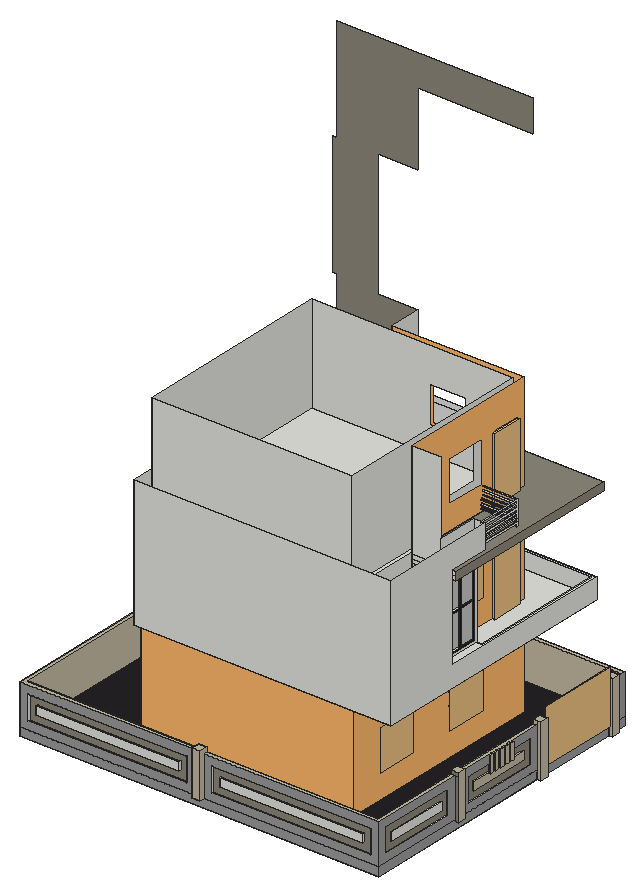
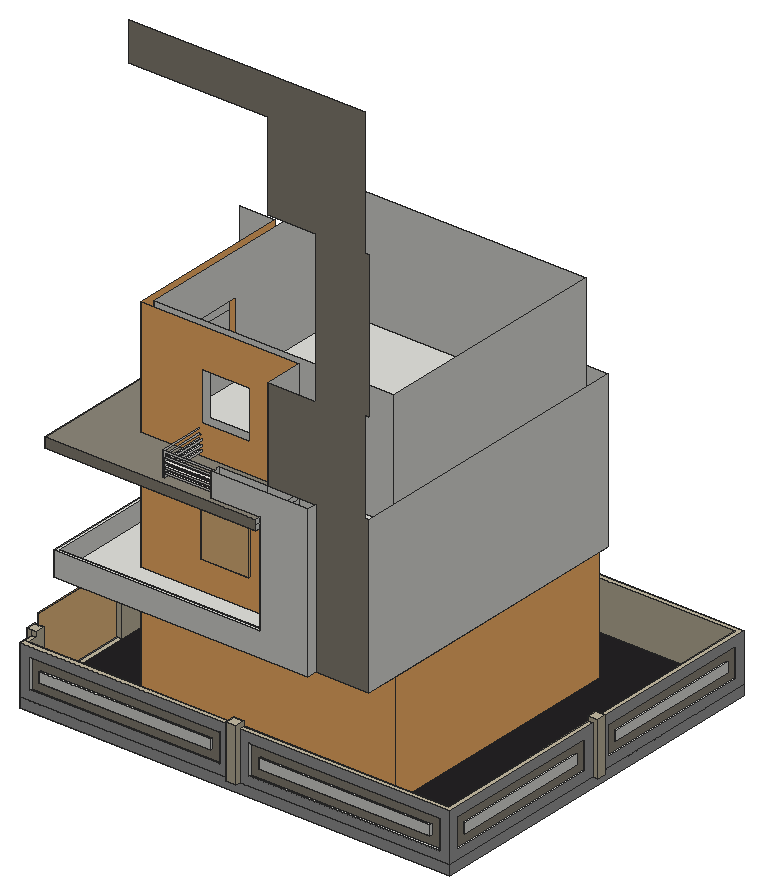
# SketchUp Ruby script. Lengths in inches.
U = 1.inch
M = Sketchup.active_model
def pt(a) = Geom::Point3d.new(a.map { |v| v * U })
def face(e, loops, mat)
  f = e.add_face(loops[0].map { |a| pt(a) })
  loops[1..].each { |l| e.add_face(l.map { |a| pt(a) }).erase! }
  f.material = f.back_material = mat if mat
  f
end
# faces: each face lists its corners as indices into pts; further lists are holes
def faces(e, pts, list, mat = nil) = list.each { |f| face(e, (f[0].is_a?(Array) ? f : [f]).map { |l| l.map { |i| pts[i] } }, mat) }
# xy, xz, yz: faces in a plane at the given z, y or x. An outline is a flat list of corners, or four numbers for a rectangle; further outlines are holes
def ring(l) = l.size == 4 ? [[l[0], l[1]], [l[2], l[1]], [l[2], l[3]], [l[0], l[3]]] : l.each_slice(2).to_a
def flat(e, list, mat, &to3) = list.each { |f| face(e, (f[0].is_a?(Array) ? f : [f]).map { |l| ring(l).map { |u, v| to3.(u, v) } }, mat) }
def xy(e, z, list, mat = nil) = flat(e, list, mat) { |x, y| [x, y, z] }
def xz(e, y, list, mat = nil) = flat(e, list, mat) { |x, z| [x, y, z] }
def yz(e, x, list, mat = nil) = flat(e, list, mat) { |y, z| [x, y, z] }
def lines(e, pts, list) = list.each { |a, b| e.add_line(pt(pts[a]), pt(pts[b])) }
# prism: a flat outline (further loops are holes) pulled along v
def prism(e, loops, v, mat = nil)
  f = face(e, loops, mat); d = Geom::Vector3d.new(v.map { |x| x * U })
  f.pushpull(f.normal.samedirection?(d) ? d.length : -d.length)
end
def box(e, o, s, mat = nil) = prism(e, [[o, [o[0] + s[0], o[1], o[2]], [o[0] + s[0], o[1] + s[1], o[2]], [o[0], o[1] + s[1], o[2]]]], [0, 0, s[2]], mat)
def at(x, y, z, deg = 0) = Geom::Transformation.translation(pt([x, y, z])) * Geom::Transformation.rotation(ORIGIN, Z_AXIS, deg.degrees)
def axes(o, x, y, z) = Geom::Transformation.new([*x, 0, *y, 0, *z, 0, *pt(o).to_a, 1])
def part(name) = M.definitions.add(name)
# library, detail: a bought-in or finely detailed component or shape, given as its bounding box
def library(name, o, s) = part(name).tap { |d| box(d.entities, o, s) }
def detail(e, o, s) = box(e.add_group.entities, o, s)
def put(e, d, t, mat = nil) = e.add_instance(d, t).tap { |i| i.material = mat if mat }
def group(e, t, mat = nil) = e.add_group.tap { |g| g.transformation = t; g.material = mat if mat }.entities
root = M.entities
M.materials.add("Brick_05_1K").color = [255, 185, 107]
M.materials.add("Brick_05_1K1").color = [195, 185, 161]
M.materials.add("Brick_09_1K").color = [135, 129, 110]
M.materials.add("M02_Ash_Whisper").color = [196, 196, 196]
M.materials.add("M08_Obsidian_Black").color = [30, 30, 30]
M.materials.add("Marble_07_1K").color = [36, 34, 36]
M.materials.add("Metal_06_1K").color = [238, 236, 231]
M.materials.add("Plaster_06_1K").color = [141, 135, 122]
M.materials.add("ThomThom - Waistcoat1").color = [155, 155, 155]
c1 = library("Modern+Gate+1",[0,0,0],[118.11,1.97,78.74])
c2 = library("mesh-164",[-1582.71,-3144.16,-23.22],[2366.42,2227.34,65.81])
c3 = part("Group13")
put(c3.entities,c2,at(294.66,859.51,3.5))
c4 = library("porta+4",[0.2,-5.42,1.33],[46.55,4.72,83.21])
xy(root,0,[[6,6,537.31,461.27]])
xy(root,0,[[537.31,299.27,543.31,311.27],[537.31,431.27,543.31,443.27]],"Brick_05_1K1")
xy(root,12,[[129.93,88.15,429.93,388.15]])
xy(root,12,[[265.65,0,277.65,6],[6,6,6,461.27,537.31,461.27,537.31,431.27,531.31,431.27,531.31,455.27,12,455.27,12,12,531.31,12,531.31,311.27,537.31,311.27,537.31,6],[537.31,146.64,543.31,158.64],[0,227.64,6,239.64],[531.31,311.27,537.31,431.27],
  [265.65,461.27,277.65,467.27]],"Brick_05_1K1")
xy(root,12,[[[12,12,531.31,455.27],[123.93,82.15,438.93,397.15]]],"Marble_07_1K")
xy(root,24,[[18,6,253.65,9],[289.65,6,525.31,9],[6,18,9,215.64],[534.31,18,537.31,134.64],[6,251.64,9,449.27],
  [18,458.27,253.65,461.27],[289.65,458.27,525.31,461.27]])
xy(root,24,[[534.31,170.64,537.31,287.27]],"Brick_05_1K1")
xy(root,36,[[30,6,241.65,9],[301.65,6,513.31,9],[6,30,9,203.64],[534.31,30,537.31,122.64],[6,263.64,9,437.27],
  [30,458.27,241.65,461.27],[301.65,458.27,513.31,461.27]])
xy(root,36,[[534.31,182.64,537.31,275.27]],"Brick_05_1K1")
xy(root,47.87,[[537.31,237.93,540.31,242.66],[537.31,247.4,540.31,252.14]],"Brick_05_1K1")
xy(root,48,[[30,6,241.65,9],[301.65,6,513.31,9],[6,30,9,203.64],[534.31,30,537.31,122.64],[6,263.64,9,437.27],
  [30,458.27,241.65,461.27],[301.65,458.27,513.31,461.27]])
xy(root,48,[[534.31,182.64,537.31,275.27],[537.31,209.5,540.31,214.24],[537.31,218.98,540.31,223.71],[537.31,228.45,540.31,233.1875]],"Brick_05_1K1")
xy(root,51,[[429.93,133.15,438.93,187.15],[429.93,262.15,438.93,316.15]])
xy(root,60,[[18,6,253.65,9],[289.65,6,525.31,9],[6,18,9,215.64],[534.31,18,537.31,134.64],[6,251.64,9,449.27],
  [18,458.27,253.65,461.27],[289.65,458.27,525.31,461.27]])
xy(root,60,[[534.31,170.64,537.31,287.27]],"Brick_05_1K1")
xy(root,72,[[6,6,265.65,6,265.65,12,12,12,12,227.64,6,227.64],[277.65,6,537.31,6,537.31,146.64,531.31,146.64,531.31,12,277.65,12],[531.31,158.64,537.31,158.64,537.31,209.5,540.31,209.5,540.31,214.24,537.31,214.24,537.31,218.98,540.31,218.98,540.31,223.71,537.31,223.71,537.31,228.45,540.31,228.45,540.31,233.1875,537.31,233.1875,537.31,237.93,540.31,237.93,540.31,242.66,537.31,242.66,537.31,247.4,540.31,247.4,540.31,252.14,537.31,252.14,537.31,299.27,531.31,299.27],[6,239.64,12,239.64,12,455.27,265.65,455.27,265.65,461.27,6,461.27],[531.31,443.27,537.31,455.27],
  [277.65,455.27,537.31,461.27]],"Brick_05_1K1")
xy(root,78,[[265.65,0,277.65,12],[531.31,146.64,543.31,158.64],[0,227.64,12,239.64],[531.31,299.27,543.31,311.27],[531.31,431.27,543.31,443.27],
  [265.65,455.27,277.65,467.27]],"Brick_05_1K1")
xy(root,105,[[429.93,133.15,438.93,187.15],[429.93,262.15,438.93,316.15]])
xy(root,156,[[117.93,76.15,117.93,82.15,438.93,82.15,438.93,397.15,117.93,397.15,117.93,445.15,183.93,445.15,183.93,457.15,498.93,457.15,498.93,76.15],[117.93,82.15,123.93,88.15],[123.93,82.15,438.93,88.15],[117.93,88.15,123.93,397.15],[123.93,88.15,129.93,397.15],
  [129.93,88.15,429.93,388.15],[429.93,88.15,438.93,397.15],[129.93,388.15,429.93,397.15]])
xy(root,162,[[132.93,91.15,429.93,388.15],[438.93,190.15,482.43,190.15,482.43,250.15,494.43,250.15,494.43,452.65,243.93,452.65,243.93,397.15,438.93,397.15]])
xy(root,165,[[429.93,346.15,438.93,382.15]])
xy(root,186,[[486.93,190.15,498.93,190.15,498.93,457.15,243.93,457.15,243.93,452.65,494.43,452.65,494.43,250.15,486.93,250.15]])
xy(root,192,[[484.46,196.15,486.93,219.15],[484.46,221.15,486.93,244.15]])
xy(root,201,[[429.93,262.15,438.93,316.15],[306.93,388.15,360.93,397.15]])
xy(root,243,[[484.46,196.15,486.93,219.15],[484.46,221.15,486.93,244.15]])
xy(root,245,[[484.46,196.15,486.93,219.15],[484.46,221.15,486.93,244.15]])
xy(root,255,[[429.93,262.15,438.93,316.15],[429.93,346.15,438.93,382.15],[306.93,388.15,360.93,397.15]])
xy(root,294,[[484.46,196.15,486.93,219.15],[484.46,221.15,486.93,244.15]])
xy(root,300,[[438.93,190.15,438.93,397.15,243.93,397.15,243.93,463.15,504.93,463.15,504.93,190.15,486.93,190.15,486.93,250.15,482.43,250.15,482.43,190.15]],"Plaster_06_1K")
xy(root,306,[[132.93,91.15,429.93,388.15]])
xy(root,312,[[132.93,91.15,429.93,388.15],[482.43,190.15,498.93,250.15],[491.43,317.65,492.93,319.15],[243.93,445.15,303.93,457.15],[363.93,449.15,366.93,453.15]])
xy(root,312,[[[438.93,190.15,482.43,190.15,482.43,250.15,498.93,250.15,498.93,190.15,504.93,190.15,504.93,463.15,243.93,463.15,243.93,457.15,303.93,457.15,303.93,445.15,243.93,445.15,243.93,397.15,438.93,397.15],[363.93,449.15,366.93,453.15],[491.43,317.65,492.93,319.15]]],"Plaster_06_1K")
xy(root,315,[[429.93,346.15,438.93,379.15],[429.93,379.15,438.93,382.15]])
xy(root,316,[[363.93,397.1,366.93,449.15],[303.93,449.15,363.93,453.15]])
xy(root,316,[[491.43,250.15,492.93,317.65],[438.93,317.65,491.43,319.15]],"Metal_06_1K")
xy(root,318,[[491.43,250.15,492.93,317.65],[438.93,317.65,491.43,319.15],[363.93,397.1,366.93,449.15],[303.93,449.15,363.93,453.15]],"Metal_06_1K")
xy(root,322,[[491.43,250.15,492.93,317.65],[438.93,317.65,491.43,319.15],[363.93,397.1,366.93,449.15],[303.93,449.15,363.93,453.15]])
xy(root,324,[[491.43,250.15,492.93,317.65],[438.93,317.65,491.43,319.15],[363.93,397.1,366.93,449.15],[303.93,449.15,363.93,453.15]],"Metal_06_1K")
xy(root,328,[[491.43,250.15,492.93,317.65],[438.93,317.65,491.43,319.15],[363.93,397.1,366.93,449.15],[303.93,449.15,363.93,453.15]])
xy(root,330,[[491.43,250.15,492.93,317.65],[438.93,317.65,491.43,319.15],[363.93,397.1,366.93,449.15],[303.93,449.15,363.93,453.15]],"Metal_06_1K")
xz(root,0,[[265.65,12,277.65,78]],"Brick_05_1K1")
xz(root,6,[[30,36,241.65,48],[301.65,36,513.31,48]])
xz(root,6,[[6,0,537.31,12],[[6,12,265.65,72],[18,24,253.65,60]],[[277.65,12,537.31,72],[289.65,24,525.31,60]]],"ThomThom - Waistcoat1")
xz(root,9,[[[18,24,253.65,60],[30,36,241.65,48]],[[289.65,24,525.31,60],[301.65,36,513.31,48]]],"Plaster_06_1K")
xz(root,12,[[12,12,12,72,265.65,72,265.65,78,277.65,78,277.65,72,531.31,72,531.31,12]],"Brick_05_1K1")
xz(root,18,[[6,24,9,60],[534.31,24,537.31,60]])
xz(root,30,[[6,36,9,48],[534.31,36,537.31,48]])
xz(root,76.15,[[117.93,156,498.93,348]])
xz(root,82.15,[[123.93,12,438.93,156]],"Brick_05_1K")
xz(root,88.15,[[129.93,12,429.93,156]])
xz(root,91.15,[[132.93,162,429.93,306],[132.93,312,429.93,456]])
xz(root,122.64,[[534.31,36,537.31,48]])
xz(root,133.15,[[429.93,51,438.93,105]])
xz(root,134.64,[[534.31,24,537.31,60]])
xz(root,146.64,[[537.31,12,543.31,72],[531.31,72,543.31,78]],"Brick_09_1K")
xz(root,158.64,[[537.31,12,543.31,72],[531.31,72,543.31,78]],"Brick_09_1K")
xz(root,170.64,[[534.31,24,537.31,60]],"Brick_05_1K1")
xz(root,182.64,[[534.31,36,537.31,48]],"Brick_05_1K1")
xz(root,187.15,[[429.93,51,438.93,105]])
xz(root,190.15,[[438.93,162,482.43,300],[482.43,186,482.43,300,438.93,300,438.93,306,498.93,306,498.93,300,486.93,300,486.93,186],[486.93,186,498.93,300],[498.93,300,504.93,306],[438.93,306,498.93,312],
  [498.93,306,504.93,312],[438.93,312,482.43,456]])
xz(root,196.15,[[484.46,192,486.93,243],[484.46,245,486.93,294]])
xz(root,203.64,[[6,36,9,48]])
xz(root,209.5,[[537.31,48,540.31,72]],"Brick_05_1K1")
xz(root,214.24,[[537.31,48,540.31,72]],"Brick_05_1K1")
xz(root,215.64,[[6,24,9,60]])
xz(root,218.98,[[537.31,48,540.31,72]],"Brick_05_1K1")
xz(root,219.15,[[484.46,192,486.93,243],[484.46,245,486.93,294]])
xz(root,221.15,[[484.46,192,486.93,243],[484.46,245,486.93,294]])
xz(root,223.71,[[537.31,48,540.31,72]],"Brick_05_1K1")
xz(root,227.64,[[0,12,6,12,6,72,12,72,12,78,0,78]],"Brick_05_1K1")
xz(root,228.45,[[537.31,48,540.31,72]],"Brick_05_1K1")
xz(root,233.1875,[[537.31,48,540.31,72]],"Brick_05_1K1")
xz(root,237.93,[[537.31,47.87,540.31,72]],"Brick_05_1K1")
xz(root,239.64,[[0,12,0,78,12,78,12,72,6,72,6,12]],"Brick_05_1K1")
xz(root,242.66,[[537.31,47.87,540.31,72]],"Brick_05_1K1")
xz(root,244.15,[[484.46,192,486.93,243],[484.46,245,486.93,294]])
xz(root,247.4,[[537.31,47.87,540.31,72]],"Brick_05_1K1")
xz(root,250.15,[[482.43,162,482.43,300,486.93,300,486.93,186,494.43,186,494.43,162],[[482.43,312,482.43,348,491.43,348,491.43,346,492.93,346,492.93,348,498.93,348,498.93,312],[491.43,340,492.93,342],[491.43,334,492.93,336],[491.43,328,492.93,330],[491.43,322,492.93,324]],[491.43,322,492.93,324],[491.43,328,492.93,330]])
xz(root,250.15,[[491.43,316,492.93,318]],"Metal_06_1K")
xz(root,251.64,[[6,24,9,60]])
xz(root,252.14,[[537.31,47.87,540.31,72]],"Brick_05_1K1")
xz(root,262.15,[[429.93,51,438.93,105],[429.93,201,438.93,255]])
xz(root,263.64,[[6,36,9,48]])
xz(root,275.27,[[534.31,36,537.31,48]],"Brick_05_1K1")
xz(root,287.27,[[534.31,24,537.31,60]],"Brick_05_1K1")
xz(root,299.27,[[537.31,0,543.31,78],[531.31,72,537.31,78]],"Brick_05_1K1")
xz(root,311.27,[[537.31,0,537.31,12,531.31,12,531.31,78,543.31,78,543.31,0]],"Brick_05_1K1")
xz(root,316.15,[[429.93,51,438.93,105],[429.93,201,438.93,255]])
xz(root,317.65,[[491.43,312,492.93,316],[491.43,318,492.93,322],[491.43,322,492.93,324],[491.43,324,492.93,328],[491.43,330,492.93,334]])
xz(root,317.65,[[438.93,316,491.43,318],[438.93,322,491.43,324],[438.93,328,491.43,330]],"Metal_06_1K")
xz(root,319.15,[[491.43,312,492.93,318],[438.93,316,491.43,318],[491.43,318,491.43,328,438.93,328,438.93,330,491.43,330,491.43,334,438.93,334,438.93,336,491.43,336,491.43,340,438.93,340,438.93,342,491.43,342,491.43,346,438.93,346,438.93,348,492.93,348,492.93,318],[438.93,322,491.43,324]],"Metal_06_1K")
xz(root,346.15,[[429.93,165,438.93,255],[429.93,315,438.93,405]])
xz(root,382.15,[[429.93,165,438.93,255],[429.93,315,438.93,405]])
xz(root,388.15,[[129.93,12,429.93,156],[[132.93,162,429.93,306],[306.93,201,360.93,255]],[[132.93,312,429.93,456],[306.93,351,360.93,405]]])
xz(root,397.1,[[363.93,316,366.93,318],[363.93,322,366.93,324],[363.93,328,366.93,330]])
xz(root,397.15,[[243.93,300,438.93,306]])
xz(root,397.15,[[123.93,12,438.93,156],[[243.93,162,438.93,300],[303.93,198,363.93,258]],[[303.93,198,363.93,258],[306.93,201,360.93,255]],[[243.93,312,438.93,456],[303.93,348,363.93,408],[363.93,340,366.93,342],[363.93,334,366.93,336]]],"Brick_05_1K")
xz(root,431.27,[[537.31,0,543.31,0,543.31,78,531.31,78,531.31,12,537.31,12]],"Brick_05_1K1")
xz(root,437.27,[[6,36,9,48]])
xz(root,443.27,[[537.31,0,543.31,78],[531.31,72,537.31,78]],"Brick_05_1K1")
xz(root,445.15,[[243.93,312,303.93,342]])
xz(root,445.15,[[117.93,156,117.93,348,123.93,348,123.93,462,117.93,462,117.93,642,123.93,642,123.93,798,414.93,798,414.93,750,243.93,750,243.93,642,183.93,642,183.93,456,243.93,456,243.93,342,183.93,342,183.93,156]],"Plaster_06_1K")
xz(root,449.15,[[363.93,312,366.93,316],[303.93,316,363.93,318],[363.93,318,366.93,322],[303.93,322,363.93,324],[363.93,324,366.93,328],
  [303.93,328,363.93,330],[363.93,330,366.93,334]])
xz(root,449.27,[[6,24,9,60]])
xz(root,452.65,[[243.93,162,494.43,186]])
xz(root,453.15,[[363.93,312,363.93,316,303.93,316,303.93,318,363.93,318,363.93,322,303.93,322,303.93,324,363.93,324,363.93,328,303.93,328,303.93,330,363.93,330,363.93,334,303.93,334,303.93,336,363.93,336,363.93,340,303.93,340,303.93,342,366.93,342,366.93,312]],"Metal_06_1K")
xz(root,455.27,[[12,12,531.31,12,531.31,72,277.65,72,277.65,78,265.65,78,265.65,72,12,72]],"Brick_05_1K1")
xz(root,457.15,[[183.93,156,183.93,342,303.93,342,303.93,312,243.93,312,243.93,186,498.93,186,498.93,156]])
xz(root,458.27,[[[18,24,253.65,60],[30,36,241.65,48]],[[289.65,24,525.31,60],[301.65,36,513.31,48]]],"Plaster_06_1K")
xz(root,461.27,[[30,36,241.65,48],[301.65,36,513.31,48]])
xz(root,461.27,[[6,0,537.31,12],[[6,12,265.65,72],[18,24,253.65,60]],[[277.65,12,537.31,72],[289.65,24,525.31,60]]],"ThomThom - Waistcoat1")
xz(root,463.15,[[243.93,300,504.93,312]],"Plaster_06_1K")
xz(root,467.27,[[265.65,12,277.65,78]],"Brick_05_1K1")
yz(root,0,[[227.64,12,239.64,78]],"Brick_05_1K1")
yz(root,6,[[30,36,203.64,48],[263.64,36,437.27,48]])
yz(root,6,[[6,0,461.27,12],[[6,12,227.64,72],[18,24,215.64,60]],[[239.64,12,461.27,72],[251.64,24,449.27,60]]],"ThomThom - Waistcoat1")
yz(root,9,[[[18,24,215.64,60],[30,36,203.64,48]],[[251.64,24,449.27,60],[263.64,36,437.27,48]]],"Plaster_06_1K")
yz(root,12,[[12,12,455.27,12,455.27,72,239.64,72,239.64,78,227.64,78,227.64,72,12,72]],"Brick_05_1K1")
yz(root,18,[[6,24,9,60],[458.27,24,461.27,60]])
yz(root,30,[[6,36,9,48],[458.27,36,461.27,48]])
yz(root,117.93,[[76.15,156,445.15,348]])
yz(root,123.93,[[82.15,12,397.15,156]],"Brick_05_1K")
yz(root,129.93,[[88.15,12,388.15,156]])
yz(root,132.93,[[91.15,162,388.15,306],[91.15,312,388.15,456]])
yz(root,183.93,[[445.15,156,457.15,342]])
yz(root,241.65,[[6,36,9,48],[458.27,36,461.27,48]])
yz(root,243.93,[[397.15,162,452.65,162,452.65,186,457.15,186,457.15,300,397.15,300],[397.15,300,457.15,306],[457.15,300,463.15,306],[397.15,306,457.15,312],[457.15,306,463.15,312],
  [397.15,312,445.15,456]])
yz(root,253.65,[[6,24,9,60],[458.27,24,461.27,60]])
yz(root,265.65,[[0,12,0,78,12,78,12,72,6,72,6,12],[461.27,12,461.27,72,455.27,72,455.27,78,467.27,78,467.27,12]],"Brick_05_1K1")
yz(root,277.65,[[0,12,6,12,6,72,12,72,12,78,0,78],[461.27,12,467.27,12,467.27,78,455.27,78,455.27,72,461.27,72]],"Brick_05_1K1")
yz(root,289.65,[[6,24,9,60],[458.27,24,461.27,60]])
yz(root,301.65,[[6,36,9,48],[458.27,36,461.27,48]])
yz(root,303.93,[[[445.15,312,457.15,312,457.15,342,453.15,342,453.15,340,449.15,340,449.15,342,445.15,342],[449.15,334,453.15,336],[449.15,328,453.15,330],[449.15,322,453.15,324],[449.15,316,453.15,318]],[449.15,316,453.15,318],[449.15,322,453.15,324],[449.15,328,453.15,330]])
yz(root,306.93,[[388.15,201,397.15,255]])
yz(root,360.93,[[388.15,201,397.15,255]])
yz(root,363.93,[[449.15,312,453.15,316],[449.15,318,453.15,322],[449.15,324,453.15,328],[449.15,330,453.15,334]])
yz(root,363.93,[[397.1,316,449.15,318],[397.1,322,449.15,324],[397.1,328,449.15,330]],"Metal_06_1K")
yz(root,366.93,[[449.15,312,453.15,312,453.15,342,397.15,342,397.15,340,449.15,340,449.15,336,397.15,336,397.15,334,449.15,334,449.15,330,397.1,330,397.1,328,449.15,328,449.15,324,397.1,324,397.1,322,449.15,322,449.15,318,397.1,318,397.1,316,449.15,316]],"Metal_06_1K")
yz(root,429.93,[[[88.15,12,388.15,156],[262.15,51,316.15,105],[133.15,51,187.15,105]],[[91.15,162,388.15,306],[346.15,165,382.15,255],[262.15,201,316.15,255]],[[91.15,312,388.15,456],[346.15,315,382.15,405],[262.15,351,316.15,405]]])
yz(root,438.93,[[[130.15,48,190.15,108],[133.15,51,187.15,105]],[[259.15,48,319.15,108],[262.15,51,316.15,105]],[[343.15,162,385.15,258],[346.15,165,382.15,255]],[[259.15,198,319.15,258],[262.15,201,316.15,255]],[190.15,300,343.15,306],
  [343.15,300,373.15,306],[373.15,300,379.15,306],[379.15,300,385.15,306],[385.15,300,388.15,306],[388.15,300,397.15,306],
  [190.15,306,343.15,312],[343.15,306,373.15,312],[373.15,306,379.15,312],[343.15,312,379.15,312,379.15,315,346.15,315,346.15,405,382.15,405,382.15,315,379.15,315,379.15,312,385.15,312,385.15,408,343.15,408],[[343.15,312,385.15,408],[346.15,315,382.15,405]],
  [317.65,322,319.15,324],[317.65,328,319.15,330]])
yz(root,438.93,[[[82.15,12,397.15,156],[259.15,48,319.15,108],[130.15,48,190.15,108]],[[190.15,162,343.15,162,343.15,258,385.15,258,385.15,162,397.15,162,397.15,300,190.15,300],[259.15,198,319.15,258]],[[190.15,312,343.15,312,343.15,408,385.15,408,385.15,312,397.15,312,397.15,456,190.15,456],[259.15,348,319.15,408],[317.65,322,319.15,324],[317.65,328,319.15,330],[317.65,334,319.15,336],[317.65,340,319.15,342]]],"Brick_05_1K")
yz(root,438.93,[[317.65,316,319.15,318]],"Metal_06_1K")
yz(root,482.43,[[190.15,162,250.15,300],[190.15,312,250.15,348]])
yz(root,484.46,[[196.15,192,219.15,243],[221.15,192,244.15,243],[196.15,245,219.15,294],[221.15,245,244.15,294]],"M02_Ash_Whisper")
yz(root,486.93,[[[190.15,186,250.15,300],[193.15,189,247.15,297]]])
yz(root,486.93,[[[193.15,189,247.15,297],[196.15,192,244.15,294]],[219.15,192,221.15,192,221.15,243,244.15,243,244.15,245,221.15,245,221.15,294,219.15,294,219.15,245,196.15,245,196.15,243,219.15,243]],"M08_Obsidian_Black")
yz(root,491.43,[[317.65,312,319.15,316],[317.65,316,319.15,318],[317.65,318,319.15,322],[250.15,322,317.65,324],[317.65,322,319.15,324],
  [317.65,324,319.15,328],[250.15,328,317.65,330],[317.65,330,319.15,334]])
yz(root,491.43,[[250.15,316,317.65,318]],"Metal_06_1K")
yz(root,492.93,[[317.65,312,319.15,312,319.15,318,250.15,318,250.15,316,317.65,316],[317.65,318,319.15,318,319.15,348,250.15,348,250.15,346,317.65,346,317.65,342,250.15,342,250.15,340,317.65,340,317.65,336,250.15,336,250.15,334,317.65,334,317.65,330,250.15,330,250.15,328,317.65,328],[250.15,322,317.65,324]],"Metal_06_1K")
yz(root,494.43,[[250.15,162,452.65,186]])
yz(root,498.93,[[76.15,156,457.15,156,457.15,186,190.15,186,190.15,312,250.15,312,250.15,348,76.15,348]])
yz(root,504.93,[[190.15,300,463.15,312]],"Plaster_06_1K")
yz(root,513.31,[[6,36,9,48],[458.27,36,461.27,48]])
yz(root,525.31,[[6,24,9,60],[458.27,24,461.27,60]])
yz(root,531.31,[[12,12,12,72,146.64,72,146.64,78,158.64,78,158.64,72,299.27,72,299.27,78,311.27,78,311.27,12],[431.27,12,431.27,78,443.27,78,443.27,72,455.27,72,455.27,12]],"Brick_05_1K1")
yz(root,534.31,[[[18,24,134.64,60],[30,36,122.64,48]],[[170.64,24,287.27,60],[182.64,36,275.27,48]]],"Plaster_06_1K")
yz(root,537.31,[[30,36,122.64,48]])
yz(root,537.31,[[431.27,0,443.27,12],[182.64,36,275.27,36,275.27,48,252.14,48,252.14,47.87,247.4,47.87,247.4,48,242.66,48,242.66,47.87,237.93,47.87,237.93,48,182.64,48],[237.93,47.87,242.66,48],[247.4,47.87,252.14,48],[209.5,48,214.24,60],
  [218.98,48,223.71,60],[228.45,48,233.1875,60],[237.93,48,242.66,60],[247.4,48,252.14,60],[214.24,60,218.98,72],
  [223.71,60,228.45,72],[233.1875,60,237.93,72],[242.66,60,247.4,72]],"Brick_05_1K1")
yz(root,537.31,[[6,0,299.27,12],[299.27,0,311.27,12],[311.27,0,431.27,12],[443.27,0,461.27,12],[[6,12,146.64,72],[18,24,134.64,60]],
  [158.64,12,299.27,12,299.27,72,252.14,72,252.14,60,287.27,60,287.27,24,170.64,24,170.64,60,209.5,60,209.5,72,158.64,72],[443.27,12,461.27,72]],"ThomThom - Waistcoat1")
yz(root,540.31,[[237.93,47.87,242.66,72],[247.4,47.87,252.14,72],[209.5,48,214.24,72],[218.98,48,223.71,72],[228.45,48,233.1875,72]],"Brick_05_1K1")
yz(root,543.31,[[299.27,0,311.27,78],[431.27,0,443.27,78],[146.64,12,158.64,78]],"Brick_05_1K1")
p = [[429.93,91.15,306],[486.93,91.15,306],[429.93,388.15,306],[438.93,388.15,306],[438.93,190.15,162],[438.93,190.15,156],
  [243.93,452.65,162],[243.93,457.15,162],[491.43,250.15,322],[491.4,250.15,322]]
lines(root,p,[[0,1],[2,3],[4,5],[6,7],[8,9]])
put(root,c1,at(537.31,431.27,12,-90))
put(root,c3,axes([440.09,286.51,109.53],[0,-0.02533,0],[0,0,0.02667],[-0.02533,0,0]))
put(root,c3,axes([440.09,157.51,109.53],[0,-0.02533,0],[0,0,0.02667],[-0.02533,0,0]))
put(root,c4,axes([444.34,385.35,160.46],[0,-1,0],[1,0,0],[0,0,1.15446]))
put(root,c3,axes([440.09,286.51,259.53],[0,-0.02533,0],[0,0,0.02667],[-0.02533,0,0]))
put(root,c3,axes([336.56,398.3125,259.53],[0.02533,0,0],[0,0,0.02667],[0,-0.02533,0]))
put(root,c4,axes([444.34,385.35,310.46],[0,-1,0],[1,0,0],[0,0,1.15446]))
